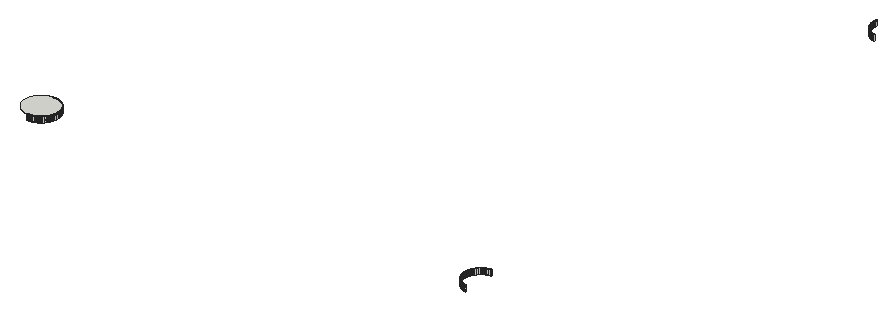
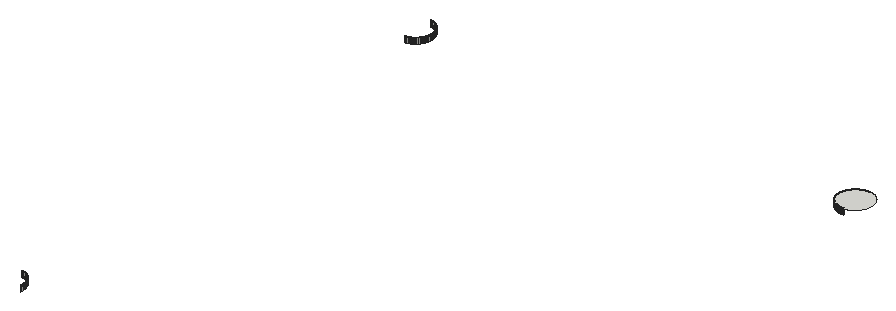
# SketchUp Ruby script. Lengths in inches.
U = 1.inch
M = Sketchup.active_model
def pt(a) = Geom::Point3d.new(a.map { |v| v * U })
def face(e, loops, mat)
  f = e.add_face(loops[0].map { |a| pt(a) })
  loops[1..].each { |l| e.add_face(l.map { |a| pt(a) }).erase! }
  f.material = f.back_material = mat if mat
  f
end
# faces: each face lists its corners as indices into pts; further lists are holes
def faces(e, pts, list, mat = nil) = list.each { |f| face(e, (f[0].is_a?(Array) ? f : [f]).map { |l| l.map { |i| pts[i] } }, mat) }
# xy, xz, yz: faces in a plane at the given z, y or x. An outline is a flat list of corners, or four numbers for a rectangle; further outlines are holes
def ring(l) = l.size == 4 ? [[l[0], l[1]], [l[2], l[1]], [l[2], l[3]], [l[0], l[3]]] : l.each_slice(2).to_a
def flat(e, list, mat, &to3) = list.each { |f| face(e, (f[0].is_a?(Array) ? f : [f]).map { |l| ring(l).map { |u, v| to3.(u, v) } }, mat) }
def xy(e, z, list, mat = nil) = flat(e, list, mat) { |x, y| [x, y, z] }
def xz(e, y, list, mat = nil) = flat(e, list, mat) { |x, z| [x, y, z] }
def yz(e, x, list, mat = nil) = flat(e, list, mat) { |y, z| [x, y, z] }
def lines(e, pts, list) = list.each { |a, b| e.add_line(pt(pts[a]), pt(pts[b])) }
# prism: a flat outline (further loops are holes) pulled along v
def prism(e, loops, v, mat = nil)
  f = face(e, loops, mat); d = Geom::Vector3d.new(v.map { |x| x * U })
  f.pushpull(f.normal.samedirection?(d) ? d.length : -d.length)
end
def box(e, o, s, mat = nil) = prism(e, [[o, [o[0] + s[0], o[1], o[2]], [o[0] + s[0], o[1] + s[1], o[2]], [o[0], o[1] + s[1], o[2]]]], [0, 0, s[2]], mat)
def at(x, y, z, deg = 0) = Geom::Transformation.translation(pt([x, y, z])) * Geom::Transformation.rotation(ORIGIN, Z_AXIS, deg.degrees)
def axes(o, x, y, z) = Geom::Transformation.new([*x, 0, *y, 0, *z, 0, *pt(o).to_a, 1])
def part(name) = M.definitions.add(name)
# library, detail: a bought-in or finely detailed component or shape, given as its bounding box
def library(name, o, s) = part(name).tap { |d| box(d.entities, o, s) }
def detail(e, o, s) = box(e.add_group.entities, o, s)
def put(e, d, t, mat = nil) = e.add_instance(d, t).tap { |i| i.material = mat if mat }
def group(e, t, mat = nil) = e.add_group.tap { |g| g.transformation = t; g.material = mat if mat }.entities
root = M.entities
xy(root,129,[[279.84,153,279.76,153.01,279.6875,153.02,279.61,153.03,279.45,153.05,279.375,153.07,279.3,153.08,279.22,153.1,279.15,153.125,279.07,153.15,279,153.17,278.92,153.2,278.71,153.29,278.64,153.33,278.57,153.36,278.43,153.44,278.37,153.48,278.3,153.53,278.24,153.57,278.17,153.62,277.93,153.82,277.88,153.88,277.82,153.93,277.62,154.17,277.57,154.24,277.53,154.3,277.48,154.37,277.44,154.43,277.36,154.57,277.33,154.64,277.29,154.71,277.2,154.92,277.17,155,277.15,155.07,277.125,155.15,277.1,155.22,277.08,155.3,277.07,155.375,277.05,155.45,277.03,155.61,277.02,155.6875,277.01,155.76,277,155.84,277,156.16,277.01,156.24,277.02,156.3125,277.03,156.39,277.05,156.55,277.07,156.625,277.08,156.7,277.1,156.78,277.125,156.85,277.15,156.93,277.17,157,277.2,157.08,277.29,157.29,277.33,157.36,277.36,157.43,277.44,157.57,277.48,157.63,277.53,157.7,277.57,157.76,277.62,157.83,277.82,158.07,277.88,158.12,277.93,158.18,278.17,158.38,278.24,158.43,278.3,158.47,278.37,158.52,278.43,158.56,278.57,158.64,278.64,158.67,278.71,158.71,278.92,158.8,279,158.83,279.07,158.85,279.15,158.875,279.22,158.9,279.3,158.92,279.375,158.93,279.45,158.95,279.61,158.97,279.6875,158.98,279.76,158.99,279.84,159,280.16,159,280.24,158.99,280.3125,158.98,280.39,158.97,280.55,158.95,280.625,158.93,280.7,158.92,280.78,158.9,280.85,158.875,280.93,158.85,281,158.83,281.08,158.8,281.29,158.71,281.36,158.67,281.43,158.64,281.57,158.56,281.63,158.52,281.7,158.47,281.76,158.43,281.83,158.38,282.07,158.18,282.12,158.12,282.18,158.07,282.38,157.83,282.43,157.76,282.47,157.7,282.52,157.63,282.56,157.57,282.64,157.43,282.67,157.36,282.71,157.29,282.8,157.08,282.83,157,282.85,156.93,282.875,156.85,282.9,156.78,282.92,156.7,282.93,156.625,282.95,156.55,282.97,156.39,282.98,156.3125,282.99,156.24,283,156.16,283,155.84,282.99,155.76,282.98,155.6875,282.97,155.61,282.95,155.45,282.93,155.375,282.92,155.3,282.9,155.22,282.875,155.15,282.85,155.07,282.83,155,282.8,154.92,282.71,154.71,282.67,154.64,282.64,154.57,282.56,154.43,282.52,154.37,282.47,154.3,282.43,154.24,282.38,154.17,282.18,153.93,282.12,153.88,282.07,153.82,281.83,153.62,281.76,153.57,281.7,153.53,281.63,153.48,281.57,153.44,281.43,153.36,281.36,153.33,281.29,153.29,281.08,153.2,281,153.17,280.93,153.15,280.85,153.125,280.78,153.1,280.7,153.08,280.625,153.07,280.55,153.05,280.39,153.03,280.3125,153.02,280.24,153.01,280.16,153]])
xz(root,153,[[279.84,128,279.92,129],[279.92,128,280,129],[280,128,280.08,129],[280.08,128,280.16,129]])
xz(root,159,[[279.84,128,279.92,129],[279.92,128,280,129],[280,128,280.08,129],[280.08,128,280.16,129]])
yz(root,283,[[155.84,128,155.92,129],[155.92,128,156,129],[156,128,156.08,129],[156.08,128,156.16,129]])
yz(root,357,[[155.84,128,155.92,129],[155.92,128,156,129],[156,128,156.08,129],[156.08,128,156.16,129],[248.84,128,248.92,129],
  [248.92,128,249,129],[249,128,249.08,129],[249.08,128,249.16,129]])
p = [[279.84,153,128],[279.76,153.01,128],[279.76,153.01,129],[279.84,153,129],[280.24,153.01,128],[280.16,153,128],
  [280.16,153,129],[280.24,153.01,129],[280.3125,153.02,128],[280.3125,153.02,129],[280.39,153.03,128],[280.39,153.03,129],
  [280.47,153.04,128],[280.47,153.04,129],[280.55,153.05,128],[280.55,153.05,129],[359.53,153.04,128],[359.45,153.05,128],
  [359.45,153.05,129],[359.53,153.04,129],[359.61,153.03,128],[359.61,153.03,129],[280.625,153.07,128],[280.625,153.07,129],
  [280.7,153.08,128],[280.7,153.08,129],[280.78,153.1,128],[280.78,153.1,129],[280.85,153.125,128],[280.85,153.125,129],
  [280.93,153.15,128],[280.93,153.15,129],[281,153.17,128],[281,153.17,129],[359.07,153.15,128],[359,153.17,128],
  [359,153.17,129],[359.07,153.15,129],[359.15,153.125,128],[359.15,153.125,129],[359.22,153.1,128],[359.22,153.1,129],
  [359.3,153.08,128],[359.3,153.08,129],[359.375,153.07,128],[359.375,153.07,129],[281.08,153.2,128],[281.08,153.2,129],
  [281.15,153.23,128],[281.15,153.23,129],[281.22,153.26,128],[281.22,153.26,129],[358.85,153.23,128],[358.78,153.26,128],
  [358.78,153.26,129],[358.85,153.23,129],[358.92,153.2,128],[358.92,153.2,129],[281.29,153.29,128],[281.29,153.29,129],
  [281.36,153.33,128],[281.36,153.33,129],[281.43,153.36,128],[281.43,153.36,129],[358.64,153.33,128],[358.57,153.36,128],
  [358.57,153.36,129],[358.64,153.33,129],[358.71,153.29,128],[358.71,153.29,129],[281.5,153.4,128],[281.5,153.4,129],
  [281.57,153.44,128],[281.57,153.44,129],[281.63,153.48,128],[281.63,153.48,129],[358.43,153.44,128],[358.37,153.48,128],
  [358.37,153.48,129],[358.43,153.44,129],[358.5,153.4,128],[358.5,153.4,129],[281.7,153.53,128],[281.7,153.53,129],
  [281.76,153.57,128],[281.76,153.57,129],[358.3,153.53,128],[358.24,153.57,128],[358.24,153.57,129],[358.3,153.53,129],
  [281.83,153.62,128],[281.83,153.62,129],[281.89,153.67,128],[281.89,153.67,129],[358.17,153.62,128],[358.11,153.67,128],
  [358.11,153.67,129],[358.17,153.62,129],[281.95,153.72,128],[281.95,153.72,129],[282.01,153.77,128],[282.01,153.77,129],
  [358.05,153.72,128],[357.99,153.77,128],[357.99,153.77,129],[358.05,153.72,129],[282.07,153.82,128],[282.07,153.82,129],
  [282.12,153.88,128],[282.12,153.88,129],[357.93,153.82,128],[357.88,153.88,128],[357.88,153.88,129],[357.93,153.82,129],
  [282.18,153.93,128],[282.18,153.93,129],[282.23,153.99,128],[282.23,153.99,129],[357.82,153.93,128],[357.77,153.99,128],
  [357.77,153.99,129],[357.82,153.93,129],[282.28,154.05,128],[282.28,154.05,129],[357.72,154.05,128],[357.72,154.05,129],
  [282.33,154.11,128],[282.33,154.11,129],[282.38,154.17,128],[282.38,154.17,129],[357.67,154.11,128],[357.62,154.17,128],
  [357.62,154.17,129],[357.67,154.11,129],[282.43,154.24,128],[282.43,154.24,129],[282.47,154.3,128],[282.47,154.3,129],
  [357.57,154.24,128],[357.53,154.3,128],[357.53,154.3,129],[357.57,154.24,129],[282.52,154.37,128],[282.52,154.37,129],
  [357.48,154.37,128],[357.48,154.37,129],[282.56,154.43,128],[282.56,154.43,129],[282.6,154.5,128],[282.6,154.5,129],
  [357.44,154.43,128],[357.4,154.5,128],[357.4,154.5,129],[357.44,154.43,129],[282.64,154.57,128],[282.64,154.57,129],
  [357.36,154.57,128],[357.36,154.57,129],[282.67,154.64,128],[282.67,154.64,129],[282.71,154.71,128],[282.71,154.71,129],
  [357.33,154.64,128],[357.29,154.71,128],[357.29,154.71,129],[357.33,154.64,129],[282.74,154.78,128],[282.74,154.78,129],
  [357.26,154.78,128],[357.26,154.78,129],[282.77,154.85,128],[282.77,154.85,129],[357.23,154.85,128],[357.23,154.85,129],
  [282.8,154.92,128],[282.8,154.92,129],[282.83,155,128],[282.83,155,129],[357.2,154.92,128],[357.17,155,128],
  [357.17,155,129],[357.2,154.92,129],[282.85,155.07,128],[282.85,155.07,129],[357.15,155.07,128],[357.15,155.07,129],
  [282.875,155.15,128],[282.875,155.15,129],[282.9,155.22,128],[282.9,155.22,129],[357.125,155.15,128],[357.1,155.22,128],
  [357.1,155.22,129],[357.125,155.15,129],[282.92,155.3,128],[282.92,155.3,129],[357.08,155.3,128],[357.08,155.3,129],
  [282.93,155.375,128],[282.93,155.375,129],[357.07,155.375,128],[357.07,155.375,129],[282.95,155.45,128],[282.95,155.45,129],
  [357.05,155.45,128],[357.05,155.45,129],[282.96,155.53,128],[282.96,155.53,129],[282.97,155.61,128],[282.97,155.61,129],
  [357.04,155.53,128],[357.03,155.61,128],[357.03,155.61,129],[357.04,155.53,129],[282.98,155.6875,128],[282.98,155.6875,129],
  [357.02,155.6875,128],[357.02,155.6875,129],[282.99,155.76,128],[282.99,155.76,129],[357.01,155.76,128],[357.01,155.76,129],
  [283,155.84,128],[283,155.84,129],[357,155.84,128],[357,155.84,129],[282.98,156.3125,128],[282.99,156.24,128],
  [282.99,156.24,129],[282.98,156.3125,129],[283,156.16,128],[283,156.16,129],[357,156.16,128],[357.01,156.24,128],
  [357.01,156.24,129],[357,156.16,129],[357.02,156.3125,128],[357.02,156.3125,129],[282.97,156.39,128],[282.97,156.39,129],
  [357.03,156.39,128],[357.03,156.39,129],[282.96,156.47,128],[282.96,156.47,129],[357.04,156.47,128],[357.04,156.47,129],
  [282.93,156.625,128],[282.95,156.55,128],[282.95,156.55,129],[282.93,156.625,129],[357.05,156.55,128],[357.05,156.55,129],
  [357.07,156.625,128],[357.07,156.625,129],[282.92,156.7,128],[282.92,156.7,129],[357.08,156.7,128],[357.08,156.7,129],
  [282.9,156.78,128],[282.9,156.78,129],[357.1,156.78,128],[357.1,156.78,129],[282.875,156.85,128],[282.875,156.85,129],
  [357.125,156.85,128],[357.125,156.85,129],[282.83,157,128],[282.85,156.93,128],[282.85,156.93,129],[282.83,157,129],
  [357.15,156.93,128],[357.15,156.93,129],[357.17,157,128],[357.17,157,129],[282.8,157.08,128],[282.8,157.08,129],
  [357.2,157.08,128],[357.2,157.08,129],[282.74,157.22,128],[282.77,157.15,128],[282.77,157.15,129],[282.74,157.22,129],
  [357.23,157.15,128],[357.23,157.15,129],[357.26,157.22,128],[357.26,157.22,129],[282.71,157.29,128],[282.71,157.29,129],
  [357.29,157.29,128],[357.29,157.29,129],[282.67,157.36,128],[282.67,157.36,129],[357.33,157.36,128],[357.33,157.36,129],
  [282.6,157.5,128],[282.64,157.43,128],[282.64,157.43,129],[282.6,157.5,129],[357.36,157.43,128],[357.36,157.43,129],
  [357.4,157.5,128],[357.4,157.5,129],[282.56,157.57,128],[282.56,157.57,129],[357.44,157.57,128],[357.44,157.57,129],
  [282.47,157.7,128],[282.52,157.63,128],[282.52,157.63,129],[282.47,157.7,129],[357.48,157.63,128],[357.48,157.63,129],
  [357.53,157.7,128],[357.53,157.7,129],[282.43,157.76,128],[282.43,157.76,129],[357.57,157.76,128],[357.57,157.76,129],
  [282.33,157.89,128],[282.38,157.83,128],[282.38,157.83,129],[282.33,157.89,129],[357.62,157.83,128],[357.62,157.83,129],
  [357.67,157.89,128],[357.67,157.89,129],[282.23,158.01,128],[282.28,157.95,128],[282.28,157.95,129],[282.23,158.01,129],
  [357.72,157.95,128],[357.72,157.95,129],[357.77,158.01,128],[357.77,158.01,129],[282.18,158.07,128],[282.18,158.07,129],
  [357.82,158.07,128],[357.82,158.07,129],[282.07,158.18,128],[282.12,158.12,128],[282.12,158.12,129],[282.07,158.18,129],
  [357.88,158.12,128],[357.88,158.12,129],[357.93,158.18,128],[357.93,158.18,129],[281.95,158.28,128],[282.01,158.23,128],
  [282.01,158.23,129],[281.95,158.28,129],[357.99,158.23,128],[357.99,158.23,129],[358.05,158.28,128],[358.05,158.28,129],
  [281.83,158.38,128],[281.89,158.33,128],[281.89,158.33,129],[281.83,158.38,129],[358.11,158.33,128],[358.11,158.33,129],
  [358.17,158.38,128],[358.17,158.38,129],[281.7,158.47,128],[281.76,158.43,128],[281.76,158.43,129],[281.7,158.47,129],
  [358.24,158.43,128],[358.24,158.43,129],[358.3,158.47,128],[358.3,158.47,129],[281.57,158.56,128],[281.63,158.52,128],
  [281.63,158.52,129],[281.57,158.56,129],[358.37,158.52,128],[358.37,158.52,129],[358.43,158.56,128],[358.43,158.56,129],
  [281.36,158.67,128],[281.43,158.64,128],[281.43,158.64,129],[281.36,158.67,129],[281.5,158.6,128],[281.5,158.6,129],
  [358.5,158.6,128],[358.5,158.6,129],[358.57,158.64,128],[358.57,158.64,129],[358.64,158.67,128],[358.64,158.67,129],
  [281.15,158.77,128],[281.22,158.74,128],[281.22,158.74,129],[281.15,158.77,129],[281.29,158.71,128],[281.29,158.71,129],
  [358.71,158.71,128],[358.71,158.71,129],[358.78,158.74,128],[358.78,158.74,129],[358.85,158.77,128],[358.85,158.77,129],
  [280.93,158.85,128],[281,158.83,128],[281,158.83,129],[280.93,158.85,129],[281.08,158.8,128],[281.08,158.8,129],
  [358.92,158.8,128],[358.92,158.8,129],[359,158.83,128],[359,158.83,129],[359.07,158.85,128],[359.07,158.85,129],
  [280.47,158.96,128],[280.55,158.95,128],[280.55,158.95,129],[280.47,158.96,129],[280.625,158.93,128],[280.625,158.93,129],
  [280.7,158.92,128],[280.7,158.92,129],[280.78,158.9,128],[280.78,158.9,129],[280.85,158.875,128],[280.85,158.875,129],
  [359.15,158.875,128],[359.15,158.875,129],[359.22,158.9,128],[359.22,158.9,129],[359.3,158.92,128],[359.3,158.92,129],
  [359.375,158.93,128],[359.375,158.93,129],[359.45,158.95,128],[359.45,158.95,129],[359.53,158.96,128],[359.53,158.96,129],
  [279.6875,158.98,128],[279.76,158.99,128],[279.76,158.99,129],[279.6875,158.98,129],[279.84,159,128],[279.84,159,129],
  [280.16,159,128],[280.24,158.99,128],[280.24,158.99,129],[280.16,159,129],[280.3125,158.98,128],[280.3125,158.98,129],
  [280.39,158.97,128],[280.39,158.97,129],[359.61,158.97,128],[359.61,158.97,129],[359.53,246.04,128],[359.45,246.05,128],
  [359.45,246.05,129],[359.53,246.04,129],[359.07,246.15,128],[359,246.17,128],[359,246.17,129],[359.07,246.15,129],
  [359.15,246.125,128],[359.15,246.125,129],[359.22,246.1,128],[359.22,246.1,129],[359.3,246.08,128],[359.3,246.08,129],
  [359.375,246.07,128],[359.375,246.07,129],[358.85,246.23,128],[358.78,246.26,128],[358.78,246.26,129],[358.85,246.23,129],
  [358.92,246.2,128],[358.92,246.2,129],[358.64,246.33,128],[358.57,246.36,128],[358.57,246.36,129],[358.64,246.33,129],
  [358.71,246.29,128],[358.71,246.29,129],[358.43,246.44,128],[358.37,246.48,128],[358.37,246.48,129],[358.43,246.44,129],
  [358.5,246.4,128],[358.5,246.4,129],[358.3,246.53,128],[358.24,246.57,128],[358.24,246.57,129],[358.3,246.53,129],
  [358.17,246.62,128],[358.11,246.67,128],[358.11,246.67,129],[358.17,246.62,129],[358.05,246.72,128],[357.99,246.77,128],
  [357.99,246.77,129],[358.05,246.72,129],[357.93,246.82,128],[357.88,246.88,128],[357.88,246.88,129],[357.93,246.82,129],
  [357.82,246.93,128],[357.77,246.99,128],[357.77,246.99,129],[357.82,246.93,129],[357.72,247.05,128],[357.72,247.05,129],
  [357.67,247.11,128],[357.62,247.17,128],[357.62,247.17,129],[357.67,247.11,129],[357.57,247.24,128],[357.53,247.3,128],
  [357.53,247.3,129],[357.57,247.24,129],[357.48,247.37,128],[357.48,247.37,129],[357.44,247.43,128],[357.4,247.5,128],
  [357.4,247.5,129],[357.44,247.43,129],[357.36,247.57,128],[357.36,247.57,129],[357.33,247.64,128],[357.29,247.71,128],
  [357.29,247.71,129],[357.33,247.64,129],[357.26,247.78,128],[357.26,247.78,129],[357.23,247.85,128],[357.23,247.85,129],
  [357.2,247.92,128],[357.17,248,128],[357.17,248,129],[357.2,247.92,129],[357.15,248.07,128],[357.15,248.07,129],
  [357.125,248.15,128],[357.1,248.22,128],[357.1,248.22,129],[357.125,248.15,129],[357.08,248.3,128],[357.08,248.3,129],
  [357.07,248.375,128],[357.07,248.375,129],[357.05,248.45,128],[357.05,248.45,129],[357.04,248.53,128],[357.03,248.61,128],
  [357.03,248.61,129],[357.04,248.53,129],[357.02,248.6875,128],[357.02,248.6875,129],[357.01,248.76,128],[357.01,248.76,129],
  [357,248.84,128],[357,248.84,129],[357,249.16,128],[357.01,249.24,128],[357.01,249.24,129],[357,249.16,129],
  [357.02,249.3125,128],[357.02,249.3125,129],[357.03,249.39,128],[357.03,249.39,129],[357.04,249.47,128],[357.04,249.47,129],
  [357.05,249.55,128],[357.05,249.55,129]]
faces(root,p,[[0,1,2,3],[4,5,6,7],[8,4,7,9],[10,8,9,11],[12,10,11,13],[14,12,13,15],[16,17,18,19],[20,16,19,21],
  [22,14,15,23],[24,22,23,25],[26,24,25,27],[28,26,27,29],[30,28,29,31],[32,30,31,33],[34,35,36,37],[38,34,37,39],
  [40,38,39,41],[42,40,41,43],[44,42,43,45],[17,44,45,18],[46,32,33,47],[48,46,47,49],[50,48,49,51],[52,53,54,55],
  [56,52,55,57],[35,56,57,36],[58,50,51,59],[60,58,59,61],[62,60,61,63],[64,65,66,67],[68,64,67,69],[53,68,69,54],
  [70,62,63,71],[72,70,71,73],[74,72,73,75],[76,77,78,79],[80,76,79,81],[65,80,81,66],[82,74,75,83],[84,82,83,85],
  [86,87,88,89],[77,86,89,78],[90,84,85,91],[92,90,91,93],[94,95,96,97],[87,94,97,88],[98,92,93,99],[100,98,99,101],
  [102,103,104,105],[95,102,105,96],[106,100,101,107],[108,106,107,109],[110,111,112,113],[103,110,113,104],[114,108,109,115],[116,114,115,117],
  [118,119,120,121],[111,118,121,112],[122,116,117,123],[119,124,125,120],[126,122,123,127],[128,126,127,129],[130,131,132,133],[124,130,133,125],
  [134,128,129,135],[136,134,135,137],[138,139,140,141],[131,138,141,132],[142,136,137,143],[139,144,145,140],[146,142,143,147],[148,146,147,149],
  [150,151,152,153],[144,150,153,145],[154,148,149,155],[151,156,157,152],[158,154,155,159],[160,158,159,161],[162,163,164,165],[156,162,165,157],
  [166,160,161,167],[163,168,169,164],[170,166,167,171],[168,172,173,169],[174,170,171,175],[176,174,175,177],[178,179,180,181],[172,178,181,173],
  [182,176,177,183],[179,184,185,180],[186,182,183,187],[188,186,187,189],[190,191,192,193],[184,190,193,185],[194,188,189,195],[191,196,197,192],
  [198,194,195,199],[196,200,201,197],[202,198,199,203],[200,204,205,201],[206,202,203,207],[208,206,207,209],[210,211,212,213],[204,210,213,205],
  [214,208,209,215],[211,216,217,212],[218,214,215,219],[216,220,221,217],[222,218,219,223],[220,224,225,221],[226,227,228,229],[227,230,231,228],
  [232,233,234,235],[233,236,237,234],[238,226,229,239],[236,240,241,237],[242,238,239,243],[240,244,245,241],[246,247,248,249],[247,242,243,248],
  [244,250,251,245],[250,252,253,251],[254,246,249,255],[252,256,257,253],[258,254,255,259],[256,260,261,257],[262,258,259,263],[260,264,265,261],
  [266,267,268,269],[267,262,263,268],[264,270,271,265],[270,272,273,271],[274,266,269,275],[272,276,277,273],[278,279,280,281],[279,274,275,280],
  [276,282,283,277],[282,284,285,283],[286,278,281,287],[284,288,289,285],[290,286,287,291],[288,292,293,289],[294,295,296,297],[295,290,291,296],
  [292,298,299,293],[298,300,301,299],[302,294,297,303],[300,304,305,301],[306,307,308,309],[307,302,303,308],[304,310,311,305],[310,312,313,311],
  [314,306,309,315],[312,316,317,313],[318,319,320,321],[319,314,315,320],[316,322,323,317],[322,324,325,323],[326,327,328,329],[327,318,321,328],
  [324,330,331,325],[330,332,333,331],[334,326,329,335],[332,336,337,333],[338,339,340,341],[339,334,335,340],[336,342,343,337],[342,344,345,343],
  [346,347,348,349],[347,338,341,348],[344,350,351,345],[350,352,353,351],[354,355,356,357],[355,346,349,356],[352,358,359,353],[358,360,361,359],
  [362,363,364,365],[363,354,357,364],[360,366,367,361],[366,368,369,367],[370,371,372,373],[371,362,365,372],[368,374,375,369],[374,376,377,375],
  [378,379,380,381],[379,382,383,380],[382,370,373,383],[376,384,385,377],[384,386,387,385],[386,388,389,387],[390,391,392,393],[391,394,395,392],
  [394,378,381,395],[388,396,397,389],[396,398,399,397],[398,400,401,399],[402,403,404,405],[403,406,407,404],[406,390,393,407],[400,408,409,401],
  [408,410,411,409],[410,412,413,411],[414,415,416,417],[415,418,419,416],[418,420,421,419],[420,422,423,421],[422,424,425,423],[424,402,405,425],
  [412,426,427,413],[426,428,429,427],[428,430,431,429],[430,432,433,431],[432,434,435,433],[434,436,437,435],[438,439,440,441],[439,442,443,440],
  [444,445,446,447],[445,448,449,446],[448,450,451,449],[450,414,417,451],[436,452,453,437],[454,455,456,457],[458,459,460,461],[462,458,461,463],
  [464,462,463,465],[466,464,465,467],[468,466,467,469],[455,468,469,456],[470,471,472,473],[474,470,473,475],[459,474,475,460],[476,477,478,479],
  [480,476,479,481],[471,480,481,472],[482,483,484,485],[486,482,485,487],[477,486,487,478],[488,489,490,491],[483,488,491,484],[492,493,494,495],
  [489,492,495,490],[496,497,498,499],[493,496,499,494],[500,501,502,503],[497,500,503,498],[504,505,506,507],[501,504,507,502],[505,508,509,506],
  [510,511,512,513],[508,510,513,509],[514,515,516,517],[511,514,517,512],[515,518,519,516],[520,521,522,523],[518,520,523,519],[521,524,525,522],
  [526,527,528,529],[524,526,529,525],[527,530,531,528],[530,532,533,531],[534,535,536,537],[532,534,537,533],[535,538,539,536],[540,541,542,543],
  [538,540,543,539],[541,544,545,542],[544,546,547,545],[546,548,549,547],[550,551,552,553],[548,550,553,549],[551,554,555,552],[554,556,557,555],
  [556,558,559,557],[560,561,562,563],[561,564,565,562],[564,566,567,565],[566,568,569,567],[568,570,571,569]])
